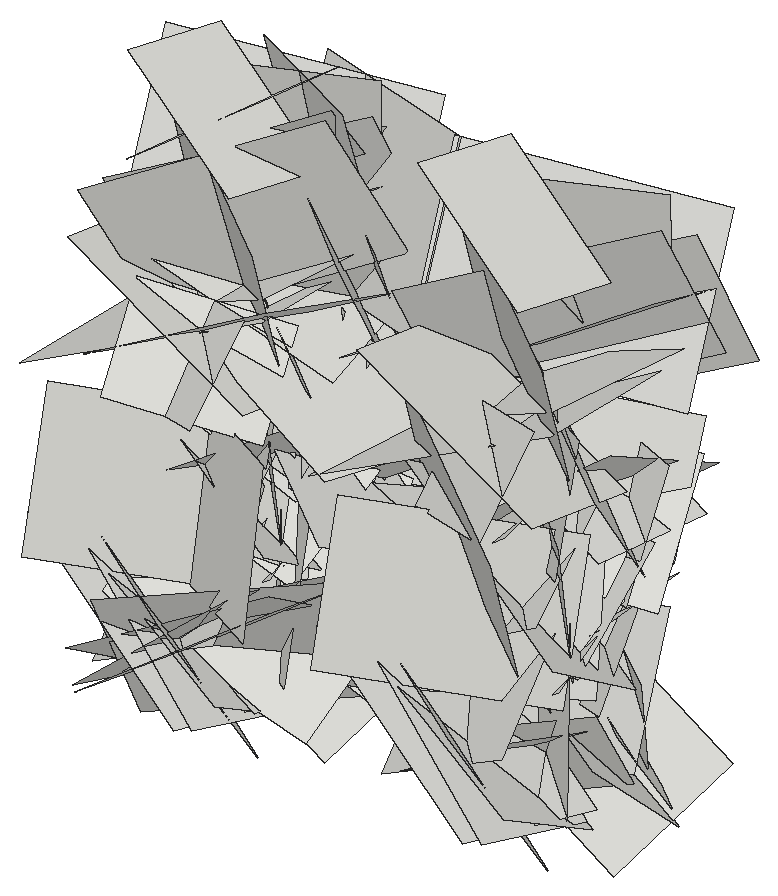
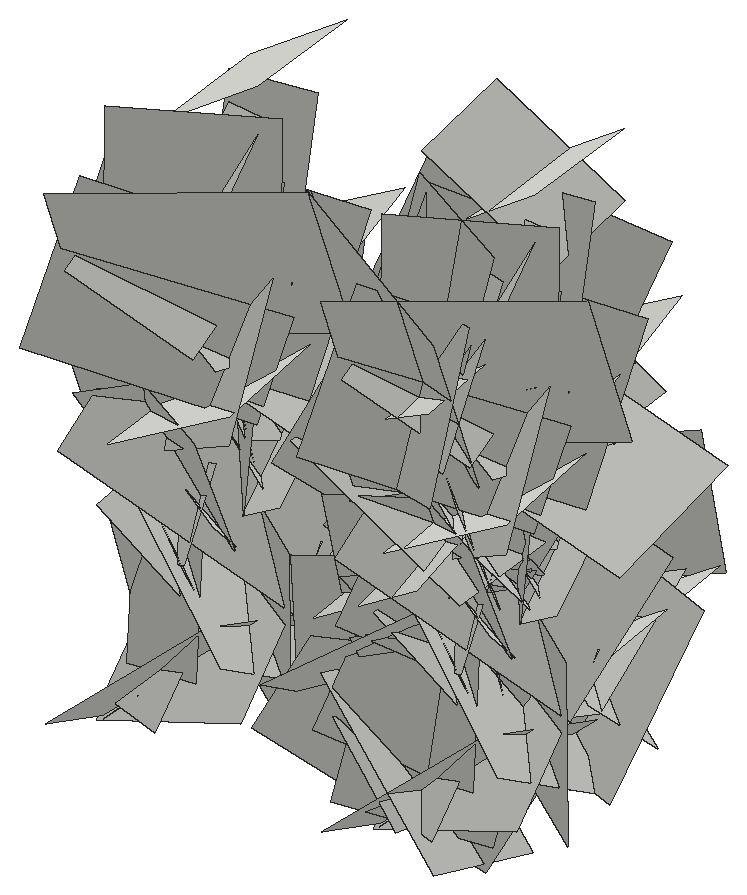
# SketchUp Ruby script. Lengths in inches.
U = 1.inch
M = Sketchup.active_model
def pt(a) = Geom::Point3d.new(a.map { |v| v * U })
def face(e, loops, mat)
  f = e.add_face(loops[0].map { |a| pt(a) })
  loops[1..].each { |l| e.add_face(l.map { |a| pt(a) }).erase! }
  f.material = f.back_material = mat if mat
  f
end
# faces: each face lists its corners as indices into pts; further lists are holes
def faces(e, pts, list, mat = nil) = list.each { |f| face(e, (f[0].is_a?(Array) ? f : [f]).map { |l| l.map { |i| pts[i] } }, mat) }
# xy, xz, yz: faces in a plane at the given z, y or x. An outline is a flat list of corners, or four numbers for a rectangle; further outlines are holes
def ring(l) = l.size == 4 ? [[l[0], l[1]], [l[2], l[1]], [l[2], l[3]], [l[0], l[3]]] : l.each_slice(2).to_a
def flat(e, list, mat, &to3) = list.each { |f| face(e, (f[0].is_a?(Array) ? f : [f]).map { |l| ring(l).map { |u, v| to3.(u, v) } }, mat) }
def xy(e, z, list, mat = nil) = flat(e, list, mat) { |x, y| [x, y, z] }
def xz(e, y, list, mat = nil) = flat(e, list, mat) { |x, z| [x, y, z] }
def yz(e, x, list, mat = nil) = flat(e, list, mat) { |y, z| [x, y, z] }
def lines(e, pts, list) = list.each { |a, b| e.add_line(pt(pts[a]), pt(pts[b])) }
# prism: a flat outline (further loops are holes) pulled along v
def prism(e, loops, v, mat = nil)
  f = face(e, loops, mat); d = Geom::Vector3d.new(v.map { |x| x * U })
  f.pushpull(f.normal.samedirection?(d) ? d.length : -d.length)
end
def box(e, o, s, mat = nil) = prism(e, [[o, [o[0] + s[0], o[1], o[2]], [o[0] + s[0], o[1] + s[1], o[2]], [o[0], o[1] + s[1], o[2]]]], [0, 0, s[2]], mat)
def at(x, y, z, deg = 0) = Geom::Transformation.translation(pt([x, y, z])) * Geom::Transformation.rotation(ORIGIN, Z_AXIS, deg.degrees)
def axes(o, x, y, z) = Geom::Transformation.new([*x, 0, *y, 0, *z, 0, *pt(o).to_a, 1])
def part(name) = M.definitions.add(name)
# library, detail: a bought-in or finely detailed component or shape, given as its bounding box
def library(name, o, s) = part(name).tap { |d| box(d.entities, o, s) }
def detail(e, o, s) = box(e.add_group.entities, o, s)
def put(e, d, t, mat = nil) = e.add_instance(d, t).tap { |i| i.material = mat if mat }
def group(e, t, mat = nil) = e.add_group.tap { |g| g.transformation = t; g.material = mat if mat }.entities
root = M.entities
c1 = part("Component\#6")
p = [[0.01,0,0],[0,3.24,4.54],[4.32,3.24,4.54],[4.33,0,0]]
faces(c1.entities,p,[[0,1,2,3]])
put(root,c1,axes([28.31,131.21,27.63],[0.2234,-0.54463,1.08834],[0.02633,1.10624,0.54877],[-1.28976,-0.07175,0.19972]))
put(root,c1,axes([14.53,134.27,30.6],[0.0256,-0.22889,-1.14247],[0.00761,-1.14266,0.22909],[1.23506,0.01178,0.02227]))
put(root,c1,axes([18.5,134.27,30.6],[-0.0256,-0.22889,-1.14247],[-0.00761,-1.14266,0.22909],[-1.23506,0.01178,0.02227]))
put(root,c1,axes([28.31,134.27,30.6],[-0.0256,-0.22889,-1.14247],[-0.00761,-1.14266,0.22909],[-1.23506,0.01178,0.02227]))
put(root,c1,axes([14.53,134.18,33.55],[-0.07538,-0.44425,-0.62436],[0.04133,-0.62833,0.44263],[0.8112,-0.00926,-0.08057]))
put(root,c1,axes([24.34,134.18,33.55],[-0.07538,-0.44425,-0.62436],[0.04133,-0.62833,0.44263],[0.8112,-0.00926,-0.08057]))
put(root,c1,axes([18.5,134.18,33.55],[0.07538,-0.44425,-0.62436],[-0.04133,-0.62833,0.44263],[-0.8112,-0.00926,-0.08057]))
put(root,c1,axes([14.53,134.17,21.91],[-0.00769,-1.04417,0.30366],[-0.13881,0.30229,1.03635],[1.14428,0.02965,0.12776]))
put(root,c1,axes([18.5,134.17,21.91],[0.00769,-1.04417,0.30366],[0.13881,0.30229,1.03635],[-1.14428,0.02965,0.12776]))
put(root,c1,axes([28.31,134.17,21.91],[0.00769,-1.04417,0.30366],[0.13881,0.30229,1.03635],[-1.14428,0.02965,0.12776]))
put(root,c1,axes([18.5,134.58,22.11],[-0.07114,-1.22092,0.271],[0.02912,0.26988,1.2227],[-1.32535,0.07146,0.01232]))
put(root,c1,axes([14.53,134.58,22.11],[0.07114,-1.22092,0.271],[-0.02912,0.26988,1.2227],[1.32535,0.07146,0.01232]))
put(root,c1,axes([28.31,134.58,22.11],[-0.07114,-1.22092,0.271],[0.02912,0.26988,1.2227],[-1.32535,0.07146,0.01232]))
put(root,c1,axes([14.53,134.42,21.5625],[-0.1234,-1.02964,0.56694],[0.11588,0.55776,1.03542],[1.24053,-0.15452,-0.04032]))
put(root,c1,axes([18.5,134.42,21.5625],[0.1234,-1.02964,0.56694],[-0.11588,0.55776,1.03542],[-1.24053,-0.15452,-0.04032]))
put(root,c1,axes([28.31,134.42,21.5625],[0.1234,-1.02964,0.56694],[-0.11588,0.55776,1.03542],[-1.24053,-0.15452,-0.04032]))
put(root,c1,axes([14.53,132.49,21.15],[0.19066,-0.73145,1.17679],[0.11238,1.19045,0.72374],[1.46442,0.00387,-0.20876]))
put(root,c1,axes([18.5,132.49,21.15],[-0.19066,-0.73145,1.17679],[-0.11238,1.19045,0.72374],[-1.46442,0.00387,-0.20876]))
put(root,c1,axes([28.31,132.49,21.15],[-0.19066,-0.73145,1.17679],[-0.11238,1.19045,0.72374],[-1.46442,0.00387,-0.20876]))
put(root,c1,axes([14.53,134.6875,22.2],[-0.10426,-0.66856,0.17597],[0.06243,0.169,0.67497],[0.73015,-0.10992,-0.03258]))
put(root,c1,axes([24.34,134.6875,22.2],[-0.10426,-0.66856,0.17597],[0.06243,0.169,0.67497],[0.73015,-0.10992,-0.03258]))
put(root,c1,axes([18.5,134.6875,22.2],[0.10426,-0.66856,0.17597],[-0.06243,0.169,0.67497],[-0.73015,-0.10992,-0.03258]))
put(root,c1,axes([14.53,131.06,25.92],[-0.11704,0.23417,0.88186],[-0.10525,0.87993,-0.24609],[0.96142,0.12483,0.08041]))
put(root,c1,axes([18.5,131.06,25.92],[0.11704,0.23417,0.88186],[0.10525,0.87993,-0.24609],[-0.96142,0.12483,0.08041]))
put(root,c1,axes([24.34,131.06,25.92],[-0.11704,0.23417,0.88186],[-0.10525,0.87993,-0.24609],[0.96142,0.12483,0.08041]))
put(root,c1,axes([14.53,130.54,25.39],[0.14552,0.87979,0.74939],[0.0105,0.75374,-0.8867],[1.22498,-0.11098,-0.08143]))
put(root,c1,axes([18.5,130.54,25.39],[-0.14552,0.87979,0.74939],[-0.0105,0.75374,-0.8867],[-1.22498,-0.11098,-0.08143]))
put(root,c1,axes([28.31,130.54,25.39],[-0.14552,0.87979,0.74939],[-0.0105,0.75374,-0.8867],[-1.22498,-0.11098,-0.08143]))
put(root,c1,axes([14.53,135.84,31.22],[-0.16391,-1.12855,0.28901],[0.13375,0.27361,1.13591],[1.2276,-0.1805,-0.08517]))
put(root,c1,axes([18.5,135.84,31.22],[0.16391,-1.12855,0.28901],[-0.13375,0.27361,1.13591],[-1.2276,-0.1805,-0.08517]))
put(root,c1,axes([28.31,135.84,31.22],[0.16391,-1.12855,0.28901],[-0.13375,0.27361,1.13591],[-1.2276,-0.1805,-0.08517]))
put(root,c1,axes([14.53,135.18,37.85],[0.05885,-0.83818,0.13983],[-0.03078,0.13818,0.83979],[0.90022,0.05952,0.01957]))
put(root,c1,axes([18.5,135.18,37.85],[-0.05885,-0.83818,0.13983],[0.03078,0.13818,0.83979],[-0.90022,0.05952,0.01957]))
put(root,c1,axes([28.31,135.18,37.85],[-0.05885,-0.83818,0.13983],[0.03078,0.13818,0.83979],[-0.90022,0.05952,0.01957]))
put(root,c1,axes([18.5,133.37,32.625],[0.2234,-0.54463,1.08834],[0.02633,1.10624,0.54877],[-1.28976,-0.07175,0.19972]))
put(root,c1,axes([14.53,133.37,32.625],[-0.2234,-0.54463,1.08834],[-0.02633,1.10624,0.54877],[1.28976,-0.07175,0.19972]))
put(root,c1,axes([28.31,133.37,32.625],[0.2234,-0.54463,1.08834],[0.02633,1.10624,0.54877],[-1.28976,-0.07175,0.19972]))
put(root,c1,axes([14.53,131.97,28.78],[0.10091,0.74431,0.53228],[-0.01265,0.53611,-0.74754],[0.96987,-0.07045,-0.06513]))
put(root,c1,axes([18.5,131.97,28.78],[-0.10091,0.74431,0.53228],[0.01265,0.53611,-0.74754],[-0.96987,-0.07045,-0.06513]))
put(root,c1,axes([28.31,131.97,28.78],[-0.10091,0.74431,0.53228],[0.01265,0.53611,-0.74754],[-0.96987,-0.07045,-0.06513]))
put(root,c1,axes([14.53,136.41,29.65],[-0.07813,-0.63244,-0.26103],[-0.10098,-0.25049,0.63382],[0.71818,-0.10402,0.06072]))
put(root,c1,axes([18.5,136.41,29.65],[0.07813,-0.63244,-0.26103],[0.10098,-0.25049,0.63382],[-0.71818,-0.10402,0.06072]))
put(root,c1,axes([24.34,136.41,29.65],[-0.07813,-0.63244,-0.26103],[-0.10098,-0.25049,0.63382],[0.71818,-0.10402,0.06072]))
put(root,c1,axes([14.53,134.54,24.9375],[0.02484,0.40022,-0.64969],[0.07983,-0.64803,-0.39648],[0.8049,0.05192,0.05937]))
put(root,c1,axes([18.5,134.54,24.9375],[-0.02484,0.40022,-0.64969],[-0.07983,-0.64803,-0.39648],[-0.8049,0.05192,0.05937]))
put(root,c1,axes([28.31,134.54,24.9375],[-0.02484,0.40022,-0.64969],[-0.07983,-0.64803,-0.39648],[-0.8049,0.05192,0.05937]))
put(root,c1,axes([14.53,136.25,25.03],[-0.1909,-1.05424,0.65515],[0.04228,0.65676,1.06778],[1.31502,-0.17416,0.06077]))
put(root,c1,axes([18.5,136.25,25.03],[0.1909,-1.05424,0.65515],[-0.04228,0.65676,1.06778],[-1.31502,-0.17416,0.06077]))
put(root,c1,axes([28.31,136.25,25.03],[0.1909,-1.05424,0.65515],[-0.04228,0.65676,1.06778],[-1.31502,-0.17416,0.06077]))
put(root,c1,axes([14.53,132.63,34.3],[0.186,1.33026,-0.17859],[0.24164,-0.20703,-1.31812],[1.40205,-0.1408,0.25087]))
put(root,c1,axes([18.5,132.63,34.3],[-0.186,1.33026,-0.17859],[-0.24164,-0.20703,-1.31812],[-1.40205,-0.1408,0.25087]))
put(root,c1,axes([28.31,132.63,34.3],[-0.186,1.33026,-0.17859],[-0.24164,-0.20703,-1.31812],[-1.40205,-0.1408,0.25087]))
put(root,c1,axes([18.5,132.79,29.8],[-0.04873,0.29435,0.84438],[0.1159,0.841,-0.28722],[-0.94075,0.08836,-0.07912]))
put(root,c1,axes([14.53,132.79,29.8],[0.04873,0.29435,0.84438],[-0.1159,0.841,-0.28722],[0.94075,0.08836,-0.07912]))
put(root,c1,axes([28.31,132.79,29.8],[-0.04873,0.29435,0.84438],[0.1159,0.841,-0.28722],[-0.94075,0.08836,-0.07912]))
put(root,c1,axes([14.53,137.68,26.93],[0.04018,-0.30696,-1.06119],[-0.15368,-1.05402,0.2997],[1.16085,-0.12891,0.07641]))
put(root,c1,axes([18.5,137.68,26.93],[-0.04018,-0.30696,-1.06119],[0.15368,-1.05402,0.2997],[-1.16085,-0.12891,0.07641]))
put(root,c1,axes([28.31,137.68,26.93],[-0.04018,-0.30696,-1.06119],[0.15368,-1.05402,0.2997],[-1.16085,-0.12891,0.07641]))
put(root,c1,axes([14.53,133.57,26.39],[-0.0097,-0.16576,1.00827],[-0.11893,1.00238,0.16377],[1.07657,0.10924,0.02717]))
put(root,c1,axes([18.5,133.57,26.39],[0.0097,-0.16576,1.00827],[0.11893,1.00238,0.16377],[-1.07657,0.10924,0.02717]))
put(root,c1,axes([28.31,133.57,26.39],[0.0097,-0.16576,1.00827],[0.11893,1.00238,0.16377],[-1.07657,0.10924,0.02717]))
put(root,c1,axes([14.53,135.55,39.48],[0.03347,0.37514,-0.47819],[-0.05412,-0.47551,-0.37641],[0.64197,-0.05964,-0.0068]))
put(root,c1,axes([24.34,135.55,39.48],[0.03347,0.37514,-0.47819],[-0.05412,-0.47551,-0.37641],[0.64197,-0.05964,-0.0068]))
put(root,c1,axes([18.5,135.55,39.48],[-0.03347,0.37514,-0.47819],[0.05412,-0.47551,-0.37641],[-0.64197,-0.05964,-0.0068]))
put(root,c1,axes([14.53,132.63,35],[-0.22269,1.01925,0.0867],[0.15354,0.11726,-1.02752],[1.07338,0.19468,0.16497]))
put(root,c1,axes([18.5,132.63,35],[0.22269,1.01925,0.0867],[-0.15354,0.11726,-1.02752],[-1.07338,0.19468,0.16497]))
put(root,c1,axes([28.31,132.63,35],[0.22269,1.01925,0.0867],[-0.15354,0.11726,-1.02752],[-1.07338,0.19468,0.16497]))
put(root,c1,axes([14.53,133.32,22.11],[0.03082,0.0656,1.39488],[-0.001,1.39518,-0.0656],[1.48021,-0.00042,-0.02909]))
put(root,c1,axes([18.5,133.32,22.11],[-0.03082,0.0656,1.39488],[0.001,1.39518,-0.0656],[-1.48021,-0.00042,-0.02909]))
put(root,c1,axes([28.31,133.32,22.11],[-0.03082,0.0656,1.39488],[0.001,1.39518,-0.0656],[-1.48021,-0.00042,-0.02909]))
put(root,c1,axes([14.53,133.77,26.39],[-0.09062,0.64279,0.71838],[0.13606,0.72237,-0.63108],[1.01272,-0.03954,0.14907]))
put(root,c1,axes([18.5,133.77,26.39],[0.09062,0.64279,0.71838],[-0.13606,0.72237,-0.63108],[-1.01272,-0.03954,0.14907]))
put(root,c1,axes([28.31,133.77,26.39],[0.09062,0.64279,0.71838],[-0.13606,0.72237,-0.63108],[-1.01272,-0.03954,0.14907]))
put(root,c1,axes([14.53,139.12,30.95],[-0.15428,-0.64193,-0.79007],[0.04846,-0.80142,0.64273],[1.07797,-0.05585,-0.14197]))
put(root,c1,axes([18.5,139.12,30.95],[0.15428,-0.64193,-0.79007],[-0.04846,-0.80142,0.64273],[-1.07797,-0.05585,-0.14197]))
put(root,c1,axes([28.31,139.12,30.95],[0.15428,-0.64193,-0.79007],[-0.04846,-0.80142,0.64273],[-1.07797,-0.05585,-0.14197]))
put(root,c1,axes([14.53,134.64,27.51],[0.11331,0.92563,-0.03565],[-0.09128,-0.0258,-0.92812],[0.97764,-0.10969,-0.08252]))
put(root,c1,axes([18.5,134.64,27.51],[-0.11331,0.92563,-0.03565],[0.09128,-0.0258,-0.92812],[-0.97764,-0.10969,-0.08252]))
put(root,c1,axes([28.31,134.64,27.51],[-0.11331,0.92563,-0.03565],[0.09128,-0.0258,-0.92812],[-0.97764,-0.10969,-0.08252]))
put(root,c1,axes([14.53,135.17,32.61],[0.12448,1.21649,-0.63228],[-0.14654,-0.62086,-1.22019],[1.44585,-0.16766,-0.06923]))
put(root,c1,axes([18.5,135.17,32.61],[-0.12448,1.21649,-0.63228],[0.14654,-0.62086,-1.22019],[-1.44585,-0.16766,-0.06923]))
put(root,c1,axes([28.31,135.17,32.61],[-0.12448,1.21649,-0.63228],[0.14654,-0.62086,-1.22019],[-1.44585,-0.16766,-0.06923]))
put(root,c1,axes([14.53,136.8125,27.97],[-0.23976,-0.84366,1.03424],[-0.08712,1.0558,0.84327],[1.41209,-0.07811,0.22763]))
put(root,c1,axes([18.5,136.8125,27.97],[0.23976,-0.84366,1.03424],[0.08712,1.0558,0.84327],[-1.41209,-0.07811,0.22763]))
put(root,c1,axes([28.31,136.8125,27.97],[0.23976,-0.84366,1.03424],[0.08712,1.0558,0.84327],[-1.41209,-0.07811,0.22763]))
put(root,c1,axes([14.53,132.97,26.35],[0.04012,1.17129,0.65858],[-0.12839,0.65914,-1.16531],[1.41857,0.02653,-0.1241]))
put(root,c1,axes([18.5,132.97,26.35],[-0.04012,1.17129,0.65858],[0.12839,0.65914,-1.16531],[-1.41857,0.02653,-0.1241]))
put(root,c1,axes([28.31,132.97,26.35],[-0.04012,1.17129,0.65858],[0.12839,0.65914,-1.16531],[-1.41857,0.02653,-0.1241]))
put(root,c1,axes([14.53,137.29,38.52],[-0.00887,0.62519,-1.13199],[-0.07674,-1.13046,-0.62381],[1.3686,-0.05933,-0.04231]))
put(root,c1,axes([18.5,137.29,38.52],[0.00887,0.62519,-1.13199],[0.07674,-1.13046,-0.62381],[-1.3686,-0.05933,-0.04231]))
put(root,c1,axes([28.31,137.29,38.52],[0.00887,0.62519,-1.13199],[0.07674,-1.13046,-0.62381],[-1.3686,-0.05933,-0.04231]))
put(root,c1,axes([14.53,134.33,29.51],[-0.0444,0.3698,0.86525],[-0.11423,0.85852,-0.37214],[0.99086,0.11554,-0.00413]))
put(root,c1,axes([18.5,134.33,29.51],[0.0444,0.3698,0.86525],[0.11423,0.85852,-0.37214],[-0.99086,0.11554,-0.00413]))
put(root,c1,axes([24.34,134.33,29.51],[-0.0444,0.3698,0.86525],[-0.11423,0.85852,-0.37214],[0.99086,0.11554,-0.00413]))
put(root,c1,axes([14.53,139.23,29.07],[-0.06497,-1.13195,0.1646],[0.10003,0.15928,1.13044],[1.20835,-0.07404,-0.08473]))
put(root,c1,axes([18.5,139.23,29.07],[0.06497,-1.13195,0.1646],[-0.10003,0.15928,1.13044],[-1.20835,-0.07404,-0.08473]))
put(root,c1,axes([28.31,139.23,29.07],[0.06497,-1.13195,0.1646],[-0.10003,0.15928,1.13044],[-1.20835,-0.07404,-0.08473]))
put(root,c1,axes([14.53,137.68,39.44],[0.12024,0.16456,-0.83242],[0.12638,-0.83458,-0.14874],[0.89051,0.09622,0.13351]))
put(root,c1,axes([18.5,137.68,39.44],[-0.12024,0.16456,-0.83242],[-0.12638,-0.83458,-0.14874],[-0.89051,0.09622,0.13351]))
put(root,c1,axes([28.31,137.68,39.44],[-0.12024,0.16456,-0.83242],[-0.12638,-0.83458,-0.14874],[-0.89051,0.09622,0.13351]))
put(root,c1,axes([18.5,138.04,20.07],[0.12016,-0.9858,0.86253],[-0.12902,0.85408,0.99214],[-1.38246,-0.16539,-0.01763]))
put(root,c1,axes([14.53,138.04,20.07],[-0.12016,-0.9858,0.86253],[0.12902,0.85408,0.99214],[1.38246,-0.16539,-0.01763]))
put(root,c1,axes([28.31,138.04,20.07],[0.12016,-0.9858,0.86253],[-0.12902,0.85408,0.99214],[-1.38246,-0.16539,-0.01763]))
put(root,c1,axes([14.53,139.13,26.61],[-0.02912,-0.4172,-0.72752],[-0.02466,-0.72725,0.41792],[0.88863,-0.03385,-0.01224]))
put(root,c1,axes([24.34,139.13,26.61],[-0.02912,-0.4172,-0.72752],[-0.02466,-0.72725,0.41792],[0.88863,-0.03385,-0.01224]))
put(root,c1,axes([18.5,139.13,26.61],[0.02912,-0.4172,-0.72752],[0.02466,-0.72725,0.41792],[-0.88863,-0.03385,-0.01224]))
put(root,c1,axes([18.5,140.34,20.98],[-0.05969,-1.08852,-0.33352],[0.17093,-0.33819,1.07653],[-1.19461,0.00599,0.1707]))
put(root,c1,axes([14.53,140.34,20.98],[0.05969,-1.08852,-0.33352],[-0.17093,-0.33819,1.07653],[1.19461,0.00599,0.1707]))
put(root,c1,axes([28.31,140.34,20.98],[-0.05969,-1.08852,-0.33352],[0.17093,-0.33819,1.07653],[-1.19461,0.00599,0.1707]))
put(root,c1,axes([14.53,137.74,29.49],[-0.05063,0.39266,-0.56355],[-0.15447,-0.55784,-0.37633],[0.71149,-0.09317,-0.12181]))
put(root,c1,axes([24.34,137.74,29.49],[-0.05063,0.39266,-0.56355],[-0.15447,-0.55784,-0.37633],[0.71149,-0.09317,-0.12181]))
put(root,c1,axes([18.5,137.74,29.49],[0.05063,0.39266,-0.56355],[0.15447,-0.55784,-0.37633],[-0.71149,-0.09317,-0.12181]))
put(root,c1,axes([14.53,135.78,27.7],[-0.08438,0.31612,0.89331],[0.15155,0.8902,-0.30228],[0.99295,-0.109,0.12205]))
put(root,c1,axes([18.5,135.78,27.7],[0.08438,0.31612,0.89331],[-0.15155,0.8902,-0.30228],[-0.99295,-0.109,0.12205]))
put(root,c1,axes([28.31,135.78,27.7],[0.08438,0.31612,0.89331],[-0.15155,0.8902,-0.30228],[-0.99295,-0.109,0.12205]))
put(root,c1,axes([18.5,140.4,37.84],[0.00777,-0.46206,-1.23937],[-0.21731,-1.22481,0.45542],[-1.38512,0.18957,-0.0784]))
put(root,c1,axes([14.53,140.4,37.84],[-0.00777,-0.46206,-1.23937],[0.21731,-1.22481,0.45542],[1.38512,0.18957,-0.0784]))
put(root,c1,axes([28.31,140.4,37.84],[0.00777,-0.46206,-1.23937],[-0.21731,-1.22481,0.45542],[-1.38512,0.18957,-0.0784]))
put(root,c1,axes([14.53,138.35,27.1],[-0.19626,0.31166,-0.79897],[0.02742,-0.81497,-0.3239],[0.90864,0.09191,-0.1628]))
put(root,c1,axes([24.34,138.35,27.1],[-0.19626,0.31166,-0.79897],[0.02742,-0.81497,-0.3239],[0.90864,0.09191,-0.1628]))
put(root,c1,axes([18.5,138.35,27.1],[0.19626,0.31166,-0.79897],[-0.02742,-0.81497,-0.3239],[-0.90864,0.09191,-0.1628]))
put(root,c1,axes([14.53,137.01,36.4],[0.10049,0.69541,-0.2411],[0.01368,-0.24463,-0.7005],[0.78006,-0.08529,0.04335]))
put(root,c1,axes([18.5,137.01,36.4],[-0.10049,0.69541,-0.2411],[-0.01368,-0.24463,-0.7005],[-0.78006,-0.08529,0.04335]))
put(root,c1,axes([28.31,137.01,36.4],[-0.10049,0.69541,-0.2411],[-0.01368,-0.24463,-0.7005],[-0.78006,-0.08529,0.04335]))
put(root,c1,axes([14.53,137.76,20.74],[0.07875,-0.43706,0.66864],[-0.02301,0.67018,0.44047],[0.84643,0.05888,-0.05024]))
put(root,c1,axes([18.5,137.76,20.74],[-0.07875,-0.43706,0.66864],[0.02301,0.67018,0.44047],[-0.84643,0.05888,-0.05024]))
put(root,c1,axes([28.31,137.76,20.74],[-0.07875,-0.43706,0.66864],[0.02301,0.67018,0.44047],[-0.84643,0.05888,-0.05024]))
put(root,c1,axes([14.53,138.81,37.71],[-0.08326,0.50336,-1.07522],[-0.02589,-1.07803,-0.50289],[1.25818,0.01113,-0.0815]))
put(root,c1,axes([18.5,138.81,37.71],[0.08326,0.50336,-1.07522],[0.02589,-1.07803,-0.50289],[-1.25818,0.01113,-0.0815]))
put(root,c1,axes([28.31,138.81,37.71],[0.08326,0.50336,-1.07522],[0.02589,-1.07803,-0.50289],[-1.25818,0.01113,-0.0815]))
put(root,c1,axes([14.53,136.62,23.89],[-0.08859,0.63974,0.04756],[-0.12242,0.03217,-0.63572],[0.66888,0.09062,-0.11005]))
put(root,c1,axes([24.34,136.62,23.89],[-0.08859,0.63974,0.04756],[-0.12242,0.03217,-0.63572],[0.66888,0.09062,-0.11005]))
put(root,c1,axes([18.5,136.62,23.89],[0.08859,0.63974,0.04756],[0.12242,0.03217,-0.63572],[-0.66888,0.09062,-0.11005]))
